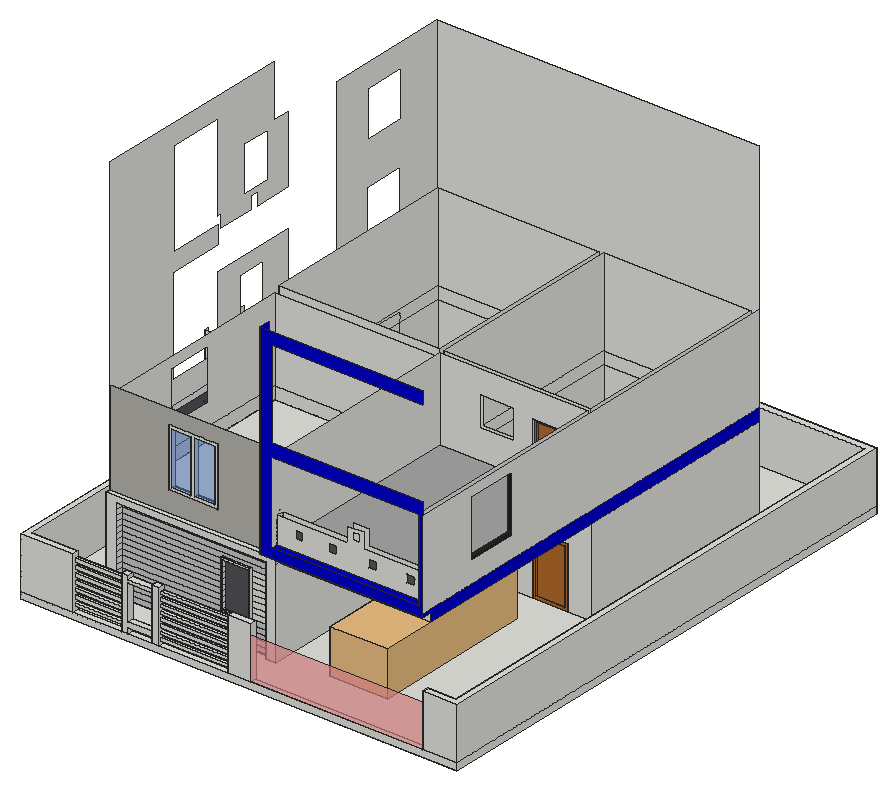
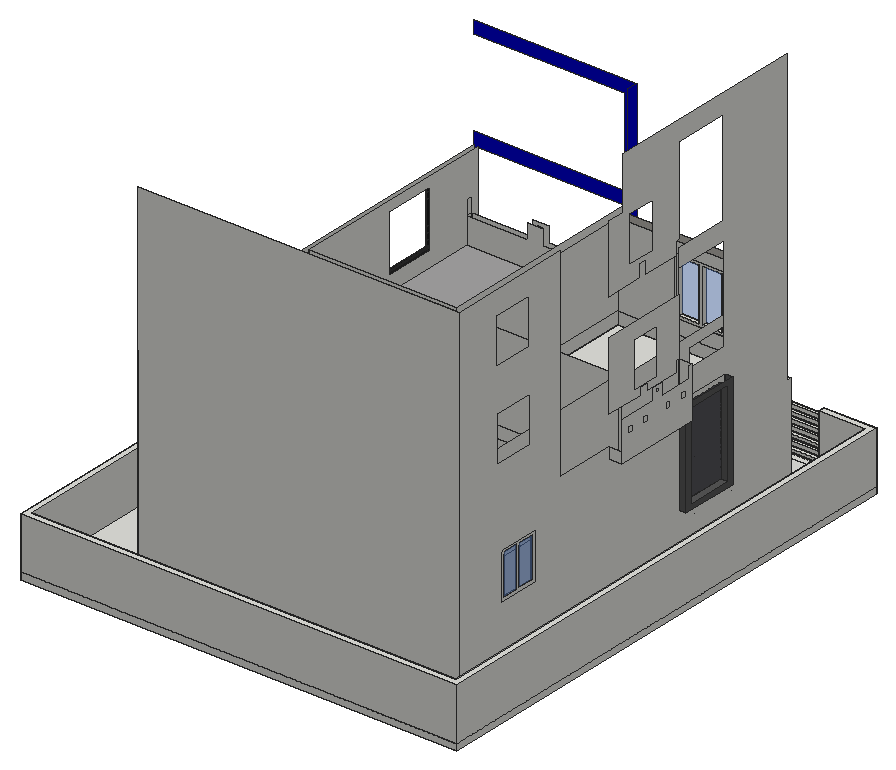
# SketchUp Ruby script. Lengths in inches.
U = 1.inch
M = Sketchup.active_model
def pt(a) = Geom::Point3d.new(a.map { |v| v * U })
def face(e, loops, mat)
  f = e.add_face(loops[0].map { |a| pt(a) })
  loops[1..].each { |l| e.add_face(l.map { |a| pt(a) }).erase! }
  f.material = f.back_material = mat if mat
  f
end
# faces: each face lists its corners as indices into pts; further lists are holes
def faces(e, pts, list, mat = nil) = list.each { |f| face(e, (f[0].is_a?(Array) ? f : [f]).map { |l| l.map { |i| pts[i] } }, mat) }
# xy, xz, yz: faces in a plane at the given z, y or x. An outline is a flat list of corners, or four numbers for a rectangle; further outlines are holes
def ring(l) = l.size == 4 ? [[l[0], l[1]], [l[2], l[1]], [l[2], l[3]], [l[0], l[3]]] : l.each_slice(2).to_a
def flat(e, list, mat, &to3) = list.each { |f| face(e, (f[0].is_a?(Array) ? f : [f]).map { |l| ring(l).map { |u, v| to3.(u, v) } }, mat) }
def xy(e, z, list, mat = nil) = flat(e, list, mat) { |x, y| [x, y, z] }
def xz(e, y, list, mat = nil) = flat(e, list, mat) { |x, z| [x, y, z] }
def yz(e, x, list, mat = nil) = flat(e, list, mat) { |y, z| [x, y, z] }
def lines(e, pts, list) = list.each { |a, b| e.add_line(pt(pts[a]), pt(pts[b])) }
# prism: a flat outline (further loops are holes) pulled along v
def prism(e, loops, v, mat = nil)
  f = face(e, loops, mat); d = Geom::Vector3d.new(v.map { |x| x * U })
  f.pushpull(f.normal.samedirection?(d) ? d.length : -d.length)
end
def box(e, o, s, mat = nil) = prism(e, [[o, [o[0] + s[0], o[1], o[2]], [o[0] + s[0], o[1] + s[1], o[2]], [o[0], o[1] + s[1], o[2]]]], [0, 0, s[2]], mat)
def at(x, y, z, deg = 0) = Geom::Transformation.translation(pt([x, y, z])) * Geom::Transformation.rotation(ORIGIN, Z_AXIS, deg.degrees)
def axes(o, x, y, z) = Geom::Transformation.new([*x, 0, *y, 0, *z, 0, *pt(o).to_a, 1])
def part(name) = M.definitions.add(name)
# library, detail: a bought-in or finely detailed component or shape, given as its bounding box
def library(name, o, s) = part(name).tap { |d| box(d.entities, o, s) }
def detail(e, o, s) = box(e.add_group.entities, o, s)
def put(e, d, t, mat = nil) = e.add_instance(d, t).tap { |i| i.material = mat if mat }
def group(e, t, mat = nil) = e.add_group.tap { |g| g.transformation = t; g.material = mat if mat }.entities
root = M.entities
M.materials.add("[Blinds Roman Hobbled Blue]").color = [81, 82, 87]
M.materials.add("[Color A02]").color = [255, 153, 153]
M.materials["[Color A02]"].alpha = 0.67
M.materials.add("[Color I06]").color = [0, 0, 204]
M.materials.add("[Color M02]").color = [198, 198, 198]
M.materials.add("[Color M06]").color = [86, 86, 86]
M.materials.add("[Color M08]").color = [30, 30, 30]
M.materials.add("[Stone Vein Gray]").color = [166, 165, 165]
M.materials.add("[Tile Travertine 2 inch]").color = [181, 178, 172]
M.materials.add("[Translucent Glass Blue]").color = [100, 149, 237]
M.materials["[Translucent Glass Blue]"].alpha = 0.5
M.materials.add("[Translucent Glass Gray]").color = [128, 128, 128]
M.materials["[Translucent Glass Gray]"].alpha = 0.5
M.materials.add("[Wood Bamboo]").color = [177, 105, 43]
c1 = library("custom el camino",[47.5625,9.86,-8],[222.64,79.59,60.9375])
c2 = part("Group\#1")
xy(c2.entities,0,[[0,0,48,1.5625],[0,1.5625,48,7.5625]],"[Wood Bamboo]")
xy(c2.entities,3.79,[[3.79,0,44.21,1.5625],[3.79,1.5625,44.21,7.5625]],"[Wood Bamboo]")
xy(c2.entities,80.21,[[3.79,0,44.21,1.5625]])
xy(c2.entities,80.21,[[3.79,1.5625,44.21,7.5625]],"[Wood Bamboo]")
xy(c2.entities,84,[[0,0,48,7.5625]],"[Wood Bamboo]")
xz(c2.entities,0,[[[0,0,48,84],[3.79,3.79,44.21,80.21]]],"[Wood Bamboo]")
xz(c2.entities,1.5625,[[3.79,3.79,44.21,80.21]],"[Wood Bamboo]")
xz(c2.entities,7.5625,[[[0,0,48,84],[3.79,3.79,44.21,80.21]],[3.79,3.79,44.21,80.21]],"[Wood Bamboo]")
yz(c2.entities,0,[[0,0,7.5625,84]],"[Wood Bamboo]")
yz(c2.entities,3.79,[[0,3.79,1.5625,80.21],[1.5625,3.79,7.5625,80.21]],"[Wood Bamboo]")
yz(c2.entities,44.21,[[0,3.79,1.5625,80.21],[1.5625,3.79,7.5625,80.21]],"[Wood Bamboo]")
yz(c2.entities,48,[[0,0,7.5625,84]],"[Wood Bamboo]")
c3 = part("Group\#4")
xy(c3.entities,0,[[0,0,32.875,4]])
xy(c3.entities,2.47,[[2.47,0,30.4,4]])
xy(c3.entities,30.4,[[2.47,0,30.4,4]])
xy(c3.entities,32.875,[[0,0,32.875,4]])
xz(c3.entities,0,[[[0,0,32.875,32.875],[2.47,2.47,30.4,30.4]]])
xz(c3.entities,0,[[2.47,2.47,30.4,30.4]],"[Translucent Glass Gray]")
xz(c3.entities,4,[[[0,0,32.875,32.875],[2.47,2.47,30.4,30.4]]])
yz(c3.entities,0,[[0,0,4,32.875]])
yz(c3.entities,2.47,[[0,2.47,4,30.4]])
yz(c3.entities,30.4,[[0,2.47,4,30.4]])
yz(c3.entities,32.875,[[0,0,4,32.875]])
c4 = part("Group\#2")
xy(c4.entities,0,[[0,0,37.8125,5]])
xy(c4.entities,2.57,[[2.57,0,17.37,5],[19.91,0,35.24,5]])
xy(c4.entities,44.8,[[2.57,0,17.37,5],[19.91,0,35.24,5]])
xy(c4.entities,47.375,[[0,0,37.8125,5]])
xz(c4.entities,0,[[[0,0,37.8125,47.375],[19.91,2.57,35.24,44.8],[2.57,2.57,17.37,44.8]]])
xz(c4.entities,0,[[2.57,2.57,17.37,44.8],[19.91,2.57,35.24,44.8]],"[Translucent Glass Blue]")
xz(c4.entities,5,[[[0,0,37.8125,47.375],[19.91,2.57,35.24,44.8],[2.57,2.57,17.37,44.8]]])
yz(c4.entities,0,[[0,0,5,47.375]])
yz(c4.entities,2.57,[[0,2.57,5,44.8]])
yz(c4.entities,17.37,[[0,2.57,5,44.8]])
yz(c4.entities,19.91,[[0,2.57,5,44.8]])
yz(c4.entities,35.24,[[0,2.57,5,44.8]])
yz(c4.entities,37.8125,[[0,0,5,47.375]])
c5 = part("Group\#3")
xy(c5.entities,0,[[0,0,37.8125,5]])
xy(c5.entities,2.57,[[2.57,0,17.37,5],[19.91,0,35.24,5]])
xy(c5.entities,44.8,[[2.57,0,17.37,5],[19.91,0,35.24,5]])
xy(c5.entities,47.375,[[0,0,37.8125,5]])
xz(c5.entities,0,[[[0,0,37.8125,47.375],[19.91,2.57,35.24,44.8],[2.57,2.57,17.37,44.8]]])
xz(c5.entities,0,[[2.57,2.57,17.37,44.8],[19.91,2.57,35.24,44.8]],"[Translucent Glass Blue]")
xz(c5.entities,5,[[[0,0,37.8125,47.375],[19.91,2.57,35.24,44.8],[2.57,2.57,17.37,44.8]]])
yz(c5.entities,0,[[0,0,5,47.375]])
yz(c5.entities,2.57,[[0,2.57,5,44.8]])
yz(c5.entities,17.37,[[0,2.57,5,44.8]])
yz(c5.entities,19.91,[[0,2.57,5,44.8]])
yz(c5.entities,35.24,[[0,2.57,5,44.8]])
yz(c5.entities,37.8125,[[0,0,5,47.375]])
xy(root,0,[[0,0,600,720]])
xy(root,9,[[0,0,0,720,600,720,600,0,552.82,0,552.82,9,591,9,591,711,9,711,9,9,72.1875,9,72.1875,0],[72.1875,0,138.87,9],[138.87,0,147.87,9],[147.87,0,180.05,9],[180.05,0,189.93,9],
  [189.93,0,285.1,9],[285.1,0,316.67,9],[316.67,0,552.82,9],[[9,9,591,711],[77.4375,49.875,77.4375,619.125,518.75,619.125,518.75,332.8125,486.18,332.8125,486.18,338.8125,438.18,338.8125,438.18,332.8125,310.75,332.8125,310.75,49.875,296.85,49.875,296.85,56.875,93.29,56.875,93.29,49.875]],[[77.4375,49.875,77.4375,619.125,518.75,619.125,518.75,332.8125,486.18,332.8125,486.18,338.8125,512.75,338.8125,512.75,613.125,310.75,613.125,310.75,338.8125,438.18,338.8125,438.18,332.8125,310.75,332.8125,310.75,49.875,296.85,49.875,296.85,56.875,93.29,56.875,93.29,49.875],[83.4375,338.8125,304.75,613.125],[83.4375,62.875,304.75,332.8125]],
  [83.4375,62.875,304.75,332.8125],[83.4375,338.8125,304.75,613.125],[310.75,338.8125,512.75,613.125]])
xy(root,14.68,[[189.54,2.77,285.1,7.27]])
xy(root,15.75,[[72.1875,2.58,142.25,7.21]])
xy(root,16.68,[[147.87,0,180,9]])
xy(root,18.49,[[189.54,2.77,285.1,7.27]])
xy(root,20.375,[[72.1875,2.58,142.25,7.21]])
xy(root,22.74,[[189.6,2.93,285.1,7.12]])
xy(root,24.37,[[147.87,0,180,9]])
xy(root,24.875,[[72.1875,2.58,138.5625,7.21]])
xy(root,26.92,[[189.6,2.93,285.1,7.12]])
xy(root,29.5,[[72.1875,2.58,138.5625,7.21]])
xy(root,30.92,[[187.85,2.93,285.1,7.12]])
xy(root,34,[[72.1875,2.58,139.25,7.21]])
xy(root,35.11,[[187.85,2.93,285.1,7.12]])
xy(root,38.625,[[72.1875,2.58,139.25,7.21]])
xy(root,39.11,[[189.85,2.93,285.1,7.12]])
xy(root,43.125,[[72.1875,2.58,139.1875,7.21]])
xy(root,43.3,[[189.85,2.93,285.1,7.12]])
xy(root,43.58,[[232.47,53.1875,272.78,56.875]])
xy(root,45.28,[[235.35,53.1875,271.02,56.875]])
xy(root,47.3,[[189.29,2.93,285.1,7.12]])
xy(root,47.75,[[72.1875,2.58,139.1875,7.21]])
xy(root,51.49,[[189.29,2.93,285.1,7.12]])
xy(root,52.25,[[72.1875,2.58,138.87,7.21]])
xy(root,54.29,[[364.5,332.8125,411.32,338.8125]])
xy(root,55.49,[[189.79,2.93,285.1,7.12]])
xy(root,56.875,[[72.1875,2.58,138.87,7.21]])
xy(root,59.375,[[67.1875,163.22,77.4375,242.75]],"[Color M06]")
xy(root,59.67,[[189.79,2.93,285.1,7.12]])
xy(root,61.375,[[72.1875,2.58,138.625,7.21]])
xy(root,63.67,[[189.93,2.93,285.1,7.12]])
xy(root,66,[[72.1875,2.58,138.625,7.21]])
xy(root,66.7,[[67.1875,170.55,77.4375,235.42]],"[Color M06]")
xy(root,67.86,[[189.93,2.93,285.1,7.12]])
xy(root,70.5,[[72.1875,2.58,138.87,7.21]])
xy(root,71.59,[[147.87,0,180.05,9]])
xy(root,71.86,[[189.35,2.93,285.1,7.12]])
xy(root,75.125,[[72.1875,2.58,138.87,7.21]])
xy(root,76.05,[[189.35,2.93,285.1,7.12]])
xy(root,76.29,[[147.87,0,180.05,9]])
xy(root,80.27,[[77.4375,489.73,83.4375,546.67]])
xy(root,81,[[0,0,72.1875,0,72.1875,9,9,9,9,711,591,711,591,9,552.82,9,552.82,0,600,0,600,720,0,720],[138.87,0,147.87,9],[180.05,0,189.93,9],[285.1,0,316.67,9]])
xy(root,93,[[438.18,332.8125,486.18,338.8125]])
xy(root,95.54,[[364.5,332.8125,411.32,338.8125]])
xy(root,108.26,[[235.35,53.1875,270.98,56.875]])
xy(root,109.97,[[232.47,53.1875,272.68,56.875]])
xy(root,123,[[83.4375,62.875,304.75,332.8125]])
xy(root,129,[[93.29,49.875,296.85,56.875],[310.75,56.875,518.75,332.8125],[83.4375,62.875,304.75,332.8125]])
xy(root,137.25,[[77.4375,49.875,310.75,56.875]])
xy(root,140.25,[[295.25,42.6875,310.75,56.875],[310.75,42.6875,518.75,56.875]])
xy(root,142.7,[[77.4375,489.73,83.4375,546.67]])
xy(root,153.3125,[[310.75,52.875,512.75,62.01]])
xy(root,153.3125,[[310.75,42.6875,512.75,52.875]],"[Color I06]")
xy(root,153.3125,[[310.75,62.01,512.75,62.01,512.75,332.8125,486.18,332.8125,486.18,338.8125,438.18,338.8125,438.18,332.8125,310.75,332.8125]],"[Stone Vein Gray]")
xy(root,164.56,[[157.85,56.875,226.03,62.875]])
xy(root,174.48,[[512.75,125.55,518.75,195.62]],"[Color M08]")
xy(root,175.33,[[59.3125,242.75,77.4375,362.77]])
xz(root,0,[[0,0,600,9],[0,9,72.1875,81],[138.87,9,147.87,9,147.87,16.68,180,16.68,180,24.37,147.87,24.37,147.87,71.59,180.05,71.59,180.05,76.29,147.87,76.29,147.87,81,138.87,81],[180.05,9,189.93,81],[285.1,9,316.67,81],
  [552.82,9,600,81]])
xz(root,0,[[316.67,9,552.82,67.52]],"[Color A02]")
xz(root,2.58,[[72.1875,15.75,142.25,20.375],[72.1875,24.875,138.5625,29.5],[72.1875,34,139.25,38.625],[72.1875,43.125,139.1875,47.75],[72.1875,52.25,138.87,56.875],
  [72.1875,61.375,138.625,66],[72.1875,70.5,138.87,75.125]])
xz(root,2.77,[[189.54,14.68,285.1,18.49]])
xz(root,2.93,[[189.6,22.74,285.1,26.92],[187.85,30.92,285.1,35.11],[189.85,39.11,285.1,43.3],[189.29,47.3,285.1,51.49],[189.79,55.49,285.1,59.67],
  [189.93,63.67,285.1,67.86],[189.35,71.86,285.1,76.05]])
xz(root,7.12,[[189.6,22.74,285.1,26.92],[187.85,30.92,285.1,35.11],[189.85,39.11,285.1,43.3],[189.29,47.3,285.1,51.49],[189.79,55.49,285.1,59.67],
  [189.93,63.67,285.1,67.86],[189.35,71.86,285.1,76.05]])
xz(root,7.21,[[72.1875,15.75,142.25,20.375],[72.1875,24.875,138.5625,29.5],[72.1875,34,139.25,38.625],[72.1875,43.125,139.1875,47.75],[72.1875,52.25,138.87,56.875],
  [72.1875,61.375,138.625,66],[72.1875,70.5,138.87,75.125]])
xz(root,7.27,[[189.54,14.68,285.1,18.49]])
xz(root,9,[[9,9,72.1875,81],[138.87,9,138.87,81,147.87,81,147.87,76.29,180.05,76.29,180.05,71.59,147.87,71.59,147.87,24.37,180,24.37,180,16.68,147.87,16.68,147.87,9],[180.05,9,189.93,81],[285.1,9,316.67,81],[552.82,9,591,81]])
xz(root,42.6875,[[[295.25,140.25,518.75,140.25,518.75,283,310.75,283,310.75,403,518.75,403,518.75,420,295.25,420],[310.75,153.3125,512.75,266]]],"[Color I06]")
xz(root,49.875,[[77.4375,9,93.29,9,93.29,129,296.85,129,296.85,9,310.75,9,310.75,137.25,77.4375,137.25]])
xz(root,52.875,[[[310.75,153.3125,512.75,153.3125,512.75,189.3125,428.93,189.3125,428.93,209.8125,408.29,209.8125,408.29,189.3125,310.75,189.3125],[335.72,169.125,346.47,179.875],[381.1,169.125,391.85,179.875],[436.72,169.125,447.47,179.875],[488.85,169.125,499.6,179.875],[414.09,194.96,423.78,205.53]]])
xz(root,52.875,[[335.72,169.125,346.47,179.875],[381.1,169.125,391.85,179.875],[436.72,169.125,447.47,179.875],[488.85,169.125,499.6,179.875]],"[Color M06]")
xz(root,53.1875,[[[232.47,43.58,272.78,43.58,272.68,46.83,272.68,109.97,232.47,109.97],[235.35,45.28,235.35,108.26,270.98,108.26,270.98,46.8,271.02,45.28]]])
xz(root,56.875,[[93.29,9,296.85,9.33],[[232.47,43.58,232.47,109.97,272.68,109.97,272.68,46.83,272.78,43.58],[235.35,45.28,271.02,45.28,270.98,46.8,270.98,108.26,235.35,108.26]],[272.68,46.83,296.85,54.33],[272.68,54.33,296.85,61.83],[272.68,61.83,296.85,69.33],
  [272.68,69.33,296.85,76.83],[272.68,76.83,296.85,84.33],[272.68,84.33,296.85,91.83],[272.68,91.83,296.85,99.33],[272.68,99.33,296.85,106.83],
  [310.75,129,518.75,140.25]])
xz(root,56.875,[[235.35,45.28,271.02,45.28,270.98,46.8,270.98,108.26,235.35,108.26]],"[Blinds Roman Hobbled Blue]")
xz(root,56.875,[[93.29,9.33,296.85,16.83],[93.29,16.83,296.85,24.33],[93.29,24.33,296.85,31.83],[93.29,31.83,296.85,39.33],[93.29,39.33,296.85,39.33,296.85,46.83,272.68,46.83,272.78,43.58,232.47,43.58,232.47,46.83,93.29,46.83],
  [93.29,46.83,232.47,54.33],[93.29,54.33,232.47,61.83],[93.29,61.83,232.47,69.33],[93.29,69.33,232.47,76.83],[93.29,76.83,232.47,84.33],
  [93.29,84.33,232.47,91.83],[93.29,91.83,232.47,99.33],[93.29,99.33,232.47,106.83],[93.29,106.83,232.47,106.83,232.47,109.97,272.68,109.97,272.68,106.83,296.85,106.83,296.85,114.33,93.29,114.33],[93.29,114.33,296.85,121.83],
  [93.29,121.83,296.85,129]],"[Color M02]")
xz(root,56.875,[[[77.4375,137.25,310.75,137.25,310.75,140.25,295.25,140.25,295.25,266,77.4375,266],[157.85,164.56,226.03,245.87]]],"[Tile Travertine 2 inch]")
xz(root,62.01,[[310.75,153.3125,310.75,189.3125,408.29,189.3125,408.29,209.8125,428.93,209.8125,428.93,189.3125,512.75,189.3125,512.75,153.3125]])
xz(root,62.875,[[83.4375,9,304.75,123],[83.4375,123,304.75,129],[83.4375,129,304.75,146],[[83.4375,146,304.75,260],[157.85,164.56,226.03,245.87]]])
xz(root,125.55,[[515.8,143.44,515.47,143.49,515.17,143.61,514.91,143.81,514.72,144.07,514.59,144.37,514.55,144.69,514.59,145.02,514.72,145.32,514.91,145.58,515.17,145.78,515.47,145.9,515.8,145.94,516.12,145.9,516.42,145.78,516.68,145.58,516.88,145.32,517.01,145.02,517.05,144.69,517.01,144.37,516.88,144.07,516.68,143.81,516.42,143.61,516.12,143.49],[515.8,151.88,515.47,151.92,515.17,152.05,514.91,152.25,514.72,152.51,514.59,152.81,514.55,153.13,514.59,153.45,514.72,153.76,514.91,154.01,515.17,154.21,515.47,154.34,515.8,154.38,516.12,154.34,516.42,154.21,516.68,154.01,516.88,153.76,517.01,153.45,517.05,153.13,517.01,152.81,516.88,152.51,516.68,152.25,516.42,152.05,516.12,151.92],[515.8,160.32,515.47,160.36,515.17,160.49,514.91,160.68,514.72,160.94,514.59,161.24,514.55,161.57,514.59,161.89,514.72,162.19,514.91,162.45,515.17,162.65,515.47,162.78,515.8,162.82,516.12,162.78,516.42,162.65,516.68,162.45,516.88,162.19,517.01,161.89,517.05,161.57,517.01,161.24,516.88,160.94,516.68,160.68,516.42,160.49,516.12,160.36],[515.8,168.76,515.47,168.8,515.17,168.92,514.91,169.12,514.72,169.38,514.59,169.68,514.55,170.01,514.59,170.33,514.72,170.63,514.91,170.89,515.17,171.09,515.47,171.21,515.8,171.26,516.12,171.21,516.42,171.09,516.68,170.89,516.88,170.63,517.01,170.33,517.05,170.01,517.01,169.68,516.88,169.38,516.68,169.12,516.42,168.92,516.12,168.8],[515.8,177.19,516.12,177.24,516.42,177.36,516.68,177.56,516.88,177.82,517.01,178.12,517.05,178.44,517.01,178.77,516.88,179.07,516.68,179.33,516.42,179.53,516.12,179.65,515.8,179.69,515.47,179.65,515.17,179.53,514.91,179.33,514.72,179.07,514.59,178.77,514.55,178.44,514.59,178.12,514.72,177.82,514.91,177.56,515.17,177.36,515.47,177.24]])
xz(root,125.55,[[[512.75,174.48,518.75,253.54],[515.8,244.69,516.12,244.74,516.42,244.86,516.68,245.06,516.88,245.32,517.01,245.62,517.05,245.94,517.01,246.27,516.88,246.57,516.68,246.83,516.42,247.03,516.12,247.15,515.8,247.19,515.47,247.15,515.17,247.03,514.91,246.83,514.72,246.57,514.59,246.27,514.55,245.94,514.59,245.62,514.72,245.32,514.91,245.06,515.17,244.86,515.47,244.74],[515.8,236.26,516.12,236.3,516.42,236.42,516.68,236.62,516.88,236.88,517.01,237.18,517.05,237.51,517.01,237.83,516.88,238.13,516.68,238.39,516.42,238.59,516.12,238.71,515.8,238.76,515.47,238.71,515.17,238.59,514.91,238.39,514.72,238.13,514.59,237.83,514.55,237.51,514.59,237.18,514.72,236.88,514.91,236.62,515.17,236.42,515.47,236.3],[515.8,227.82,516.12,227.86,516.42,227.99,516.68,228.18,516.88,228.44,517.01,228.74,517.05,229.07,517.01,229.39,516.88,229.69,516.68,229.95,516.42,230.15,516.12,230.28,515.8,230.32,515.47,230.28,515.17,230.15,514.91,229.95,514.72,229.69,514.59,229.39,514.55,229.07,514.59,228.74,514.72,228.44,514.91,228.18,515.17,227.99,515.47,227.86],[515.8,219.38,516.12,219.42,516.42,219.55,516.68,219.75,516.88,220.01,517.01,220.31,517.05,220.63,517.01,220.95,516.88,221.26,516.68,221.51,516.42,221.71,516.12,221.84,515.8,221.88,515.47,221.84,515.17,221.71,514.91,221.51,514.72,221.26,514.59,220.95,514.55,220.63,514.59,220.31,514.72,220.01,514.91,219.75,515.17,219.55,515.47,219.42],[515.8,210.94,516.12,210.99,516.42,211.11,516.68,211.31,516.88,211.57,517.01,211.87,517.05,212.19,517.01,212.52,516.88,212.82,516.68,213.08,516.42,213.28,516.12,213.4,515.8,213.44,515.47,213.4,515.17,213.28,514.91,213.08,514.72,212.82,514.59,212.52,514.55,212.19,514.59,211.87,514.72,211.57,514.91,211.31,515.17,211.11,515.47,210.99],[515.8,202.51,516.12,202.55,516.42,202.67,516.68,202.87,516.88,203.13,517.01,203.43,517.05,203.76,517.01,204.08,516.88,204.38,516.68,204.64,516.42,204.84,516.12,204.96,515.8,205.01,515.47,204.96,515.17,204.84,514.91,204.64,514.72,204.38,514.59,204.08,514.55,203.76,514.59,203.43,514.72,203.13,514.91,202.87,515.17,202.67,515.47,202.55],[515.8,194.07,516.12,194.11,516.42,194.24,516.68,194.43,516.88,194.69,517.01,194.99,517.05,195.32,517.01,195.64,516.88,195.94,516.68,196.2,516.42,196.4,516.12,196.53,515.8,196.57,515.47,196.53,515.17,196.4,514.91,196.2,514.72,195.94,514.59,195.64,514.55,195.32,514.59,194.99,514.72,194.69,514.91,194.43,515.17,194.24,515.47,194.11],[515.8,185.63,516.12,185.67,516.42,185.8,516.68,186,516.88,186.26,517.01,186.56,517.05,186.88,517.01,187.2,516.88,187.51,516.68,187.76,516.42,187.96,516.12,188.09,515.8,188.13,515.47,188.09,515.17,187.96,514.91,187.76,514.72,187.51,514.59,187.2,514.55,186.88,514.59,186.56,514.72,186.26,514.91,186,515.17,185.8,515.47,185.67],[515.8,177.19,516.12,177.24,516.42,177.36,516.68,177.56,516.88,177.82,517.01,178.12,517.05,178.44,517.01,178.77,516.88,179.07,516.68,179.33,516.42,179.53,516.12,179.65,515.8,179.69,515.47,179.65,515.17,179.53,514.91,179.33,514.72,179.07,514.59,178.77,514.55,178.44,514.59,178.12,514.72,177.82,514.91,177.56,515.17,177.36,515.47,177.24]]],"[Color M08]")
xz(root,163.22,[[67.1875,59.375,77.4375,192.66]],"[Color M06]")
xz(root,170.55,[[67.1875,66.7,77.4375,185.33]],"[Color M06]")
xz(root,195.62,[[[512.75,174.48,518.75,253.54],[515.8,244.69,515.47,244.74,515.17,244.86,514.91,245.06,514.72,245.32,514.59,245.62,514.55,245.94,514.59,246.27,514.72,246.57,514.91,246.83,515.17,247.03,515.47,247.15,515.8,247.19,516.12,247.15,516.42,247.03,516.68,246.83,516.88,246.57,517.01,246.27,517.05,245.94,517.01,245.62,516.88,245.32,516.68,245.06,516.42,244.86,516.12,244.74],[515.8,236.26,515.47,236.3,515.17,236.42,514.91,236.62,514.72,236.88,514.59,237.18,514.55,237.51,514.59,237.83,514.72,238.13,514.91,238.39,515.17,238.59,515.47,238.71,515.8,238.76,516.12,238.71,516.42,238.59,516.68,238.39,516.88,238.13,517.01,237.83,517.05,237.51,517.01,237.18,516.88,236.88,516.68,236.62,516.42,236.42,516.12,236.3],[515.8,194.07,515.47,194.11,515.17,194.24,514.91,194.43,514.72,194.69,514.59,194.99,514.55,195.32,514.59,195.64,514.72,195.94,514.91,196.2,515.17,196.4,515.47,196.53,515.8,196.57,516.12,196.53,516.42,196.4,516.68,196.2,516.88,195.94,517.01,195.64,517.05,195.32,517.01,194.99,516.88,194.69,516.68,194.43,516.42,194.24,516.12,194.11],[515.8,210.94,515.47,210.99,515.17,211.11,514.91,211.31,514.72,211.57,514.59,211.87,514.55,212.19,514.59,212.52,514.72,212.82,514.91,213.08,515.17,213.28,515.47,213.4,515.8,213.44,516.12,213.4,516.42,213.28,516.68,213.08,516.88,212.82,517.01,212.52,517.05,212.19,517.01,211.87,516.88,211.57,516.68,211.31,516.42,211.11,516.12,210.99]]],"[Color M08]")
xz(root,196.24,[[515.8,177.19,515.47,177.24,515.17,177.36,514.91,177.56,514.72,177.82,514.59,178.12,514.55,178.44,514.59,178.77,514.72,179.07,514.91,179.33,515.17,179.53,515.47,179.65,515.8,179.69,516.12,179.65,516.42,179.53,516.68,179.33,516.88,179.07,517.01,178.77,517.05,178.44,517.01,178.12,516.88,177.82,516.68,177.56,516.42,177.36,516.12,177.24]])
xz(root,235.42,[[67.1875,66.7,77.4375,185.33]],"[Color M06]")
xz(root,242.75,[[59.3125,175.33,67.1875,175.33,67.1875,192.66,77.4375,192.66,77.4375,246.02,59.3125,246.02],[67.1875,175.33,77.4375,192.66]])
xz(root,242.75,[[67.1875,59.375,77.4375,175.33]],"[Color M06]")
xz(root,332.8125,[[83.4375,9,304.75,123],[[310.75,9,438.18,9,438.18,93,486.18,93,486.18,9,518.75,9,518.75,129,310.75,129],[364.5,54.29,411.32,95.54]],[83.4375,123,194.09,129],[194.09,123,222.91,129],[222.91,123,304.75,129],
  [83.4375,129,304.75,146],[83.4375,146,304.75,260],[[310.75,153.3125,438.18,153.3125,438.18,230,486.18,230,486.18,153.3125,512.75,153.3125,512.75,266,310.75,266],[364.5,192.97,411.32,234.22]]])
xz(root,338.8125,[[83.4375,9,304.75,129],[[310.75,9,310.75,129,512.75,129,512.75,9,486.18,9,486.18,93,438.18,93,438.18,9],[364.5,54.29,411.32,95.54]],[83.4375,129,304.75,146],[310.75,129,310.75,146,438.18,146,438.18,153.3125,486.18,153.3125,486.18,146,512.75,146,512.75,129],[83.4375,146,304.75,266],
  [[310.75,146,310.75,266,512.75,266,512.75,146,486.18,146,486.18,230,438.18,230,438.18,146],[364.5,192.97,411.32,234.22]]])
xz(root,362.77,[[59.3125,175.33,77.4375,190.375]])
xz(root,489.73,[[77.4375,80.27,83.4375,142.7]])
xz(root,546.67,[[77.4375,80.27,83.4375,142.7]])
xz(root,613.125,[[83.4375,9,304.75,129],[310.75,9,512.75,129],[83.4375,129,304.75,146],[310.75,129,512.75,146],[83.4375,146,304.75,266],
  [310.75,146,512.75,266]])
xz(root,619.125,[[77.4375,9,518.75,468]])
xz(root,711,[[9,9,591,81]])
xz(root,720,[[0,0,600,9],[0,9,600,81]])
yz(root,0,[[0,0,720,9],[0,9,720,81]])
yz(root,9,[[9,9,711,81]])
yz(root,59.3125,[[[242.75,175.33,242.75,246.02,248.07,246.02,248.07,230.24,294.97,229.95,294.97,246.02,309.77,246.02,309.77,229.95,362.77,230.24,362.77,175.33],[344.8125,208.79,353.375,217.35],[318.6875,208.79,327.25,217.35],[279.625,208.79,288.1875,217.35],[253.3125,209.47,261.875,218.03],[300.15,237.48,305.34,242.66]]])
yz(root,67.1875,[[[163.22,59.375,242.75,192.66],[170.55,66.7,235.42,185.33]]],"[Color M06]")
yz(root,72.1875,[[[0,9,9,81],[2.58,70.5,7.21,75.125],[2.58,61.375,7.21,66],[2.58,52.25,7.21,56.875],[2.58,43.125,7.21,47.75],[2.58,34,7.21,38.625],[2.58,24.875,7.21,29.5],[2.58,15.75,7.21,20.375]]])
yz(root,77.4375,[[[49.875,9,49.875,137.25,56.875,137.25,56.875,540,338.8125,540,338.8125,468,362.77,468,362.77,375.04,311.55,375.04,311.55,392.36,298.6,392.36,298.6,375.04,248.07,375.04,248.07,392.36,241.87,392.36,241.87,512.67,166.06,512.67,166.06,382.11,241.6875,382.11,241.6875,356.84,164.28,356.84,164.28,225.6875,241.6875,225.6875,241.6875,323.97,362.77,323.97,362.77,230.24,309.77,229.95,309.77,246.02,294.97,246.02,294.97,229.95,248.07,230.24,248.07,246.02,242.75,246.02,242.75,192.66,163.22,192.66,163.22,59.375,242.75,59.375,242.75,175.33,362.77,175.33,362.77,190.375,446.27,190.375,446.27,468,619.125,468,619.125,9],[498.5625,252.44,555.5,314.88],[500.02,373.64,556.96,436.08],[489.73,80.27,546.67,142.7],[287.71,398.88,327.77,461.44],[279.8125,240.34,319.875,302.91]],[[163.22,59.375,242.75,192.66],[170.55,66.7,235.42,185.33]]])
yz(root,77.4375,[[170.55,66.7,235.42,185.33]],"[Blinds Roman Hobbled Blue]")
yz(root,83.4375,[[62.875,9,332.8125,123],[338.8125,9,613.125,9,613.125,129,546.67,129,546.67,80.27,489.73,80.27,489.73,129,338.8125,129],[489.73,80.27,546.67,129],[62.875,123,332.8125,129],[62.875,129,332.8125,146],
  [338.8125,129,489.73,129,489.73,142.7,546.67,142.7,546.67,129,613.125,129,613.125,146,338.8125,146],[489.73,129,546.67,142.7],[[62.875,146,332.8125,260],[153.86,176.04,217.18,245.85]],[338.8125,146,613.125,266]])
yz(root,93.29,[[49.875,9,56.875,9.33],[49.875,9.33,56.875,16.83],[49.875,16.83,56.875,24.33],[49.875,24.33,56.875,31.83],[49.875,31.83,56.875,39.33],
  [49.875,39.33,56.875,46.83],[49.875,46.83,56.875,54.33],[49.875,54.33,56.875,61.83],[49.875,61.83,56.875,69.33],[49.875,69.33,56.875,76.83],
  [49.875,76.83,56.875,84.33],[49.875,84.33,56.875,91.83],[49.875,91.83,56.875,99.33],[49.875,99.33,56.875,106.83],[49.875,106.83,56.875,114.33],
  [49.875,114.33,56.875,121.83],[49.875,121.83,56.875,129]])
yz(root,138.5625,[[2.58,24.875,7.21,29.5]])
yz(root,138.625,[[2.58,61.375,7.21,66]])
yz(root,138.87,[[[0,9,9,81],[2.58,70.5,7.21,75.125],[2.58,52.25,7.21,56.875]]])
yz(root,139.1875,[[2.58,43.125,7.21,47.75]])
yz(root,139.25,[[2.58,34,7.21,38.625]])
yz(root,142.25,[[2.58,15.75,7.21,20.375]])
yz(root,147.87,[[0,9,9,16.68],[0,24.37,9,71.59],[0,76.29,9,81]])
yz(root,157.85,[[56.875,164.56,62.875,245.87]])
yz(root,180,[[0,16.68,9,24.37]])
yz(root,180.05,[[0,9,9,71.59],[0,71.59,9,76.29],[0,76.29,9,81]])
yz(root,187.85,[[2.93,30.92,7.12,35.11]])
yz(root,189.29,[[2.93,47.3,7.12,51.49]])
yz(root,189.35,[[2.93,71.86,7.12,76.05]])
yz(root,189.54,[[2.77,14.68,7.27,18.49]])
yz(root,189.6,[[2.93,22.74,7.12,26.92]])
yz(root,189.79,[[2.93,55.49,7.12,59.67]])
yz(root,189.85,[[2.93,39.11,7.12,43.3]])
yz(root,189.93,[[[0,9,9,81],[2.93,63.67,7.12,67.86]]])
yz(root,226.03,[[56.875,164.56,62.875,245.87]])
yz(root,232.47,[[53.1875,43.58,56.875,109.97]])
yz(root,235.35,[[53.1875,45.28,56.875,46.83],[53.1875,46.83,56.875,54.33],[53.1875,54.33,56.875,61.83],[53.1875,61.83,56.875,69.33],[53.1875,69.33,56.875,76.83],
  [53.1875,76.83,56.875,84.33],[53.1875,84.33,56.875,91.83],[53.1875,91.83,56.875,99.33],[53.1875,99.33,56.875,106.83],[53.1875,106.83,56.875,108.26]])
yz(root,270.98,[[53.1875,46.8,56.875,106.83],[53.1875,106.83,56.875,108.26]])
yz(root,272.68,[[53.1875,46.83,56.875,109.97]])
yz(root,285.1,[[[0,9,9,81],[2.93,71.86,7.12,76.05],[2.93,63.67,7.12,67.86],[2.93,55.49,7.12,59.67],[2.93,47.3,7.12,51.49],[2.93,39.11,7.12,43.3],[2.93,30.92,7.12,35.11],[2.93,22.74,7.12,26.92],[2.77,14.68,7.27,18.49]]])
yz(root,295.25,[[42.6875,140.25,56.875,420]],"[Color I06]")
yz(root,296.85,[[49.875,9,56.875,9.33],[49.875,9.33,56.875,129]])
yz(root,304.75,[[62.875,9,332.8125,123],[338.8125,9,613.125,129],[62.875,123,332.8125,129],[62.875,129,332.8125,146],[338.8125,129,613.125,146],
  [62.875,146,332.8125,260],[338.8125,146,613.125,266]])
yz(root,310.75,[[49.875,9,332.8125,129],[338.8125,9,613.125,129],[49.875,129,56.875,137.25],[338.8125,129,613.125,146],[338.8125,146,613.125,266],
  [[42.6875,153.3125,52.875,153.3125,52.875,189.3125,62.01,189.3125,62.01,153.3125,332.8125,153.3125,332.8125,266,42.6875,266],[56.1,191.91,59.54,195.34]],[52.875,153.3125,62.01,189.3125]])
yz(root,316.67,[[0,9,9,81]])
yz(root,364.5,[[332.8125,54.29,338.8125,95.54]])
yz(root,411.32,[[332.8125,54.29,338.8125,95.54]])
yz(root,438.18,[[332.8125,9,338.8125,93],[332.8125,153.3125,338.8125,230]])
yz(root,486.18,[[332.8125,9,338.8125,93],[332.8125,153.3125,338.8125,230]])
yz(root,512.75,[[338.8125,9,613.125,129],[338.8125,129,613.125,146],[338.8125,146,613.125,266],[[42.6875,153.3125,42.6875,266,332.8125,266,332.8125,153.3125,62.01,153.3125,62.01,189.3125,62.375,209.8125,52.875,209.8125,52.875,153.3125],[125.55,174.48,195.62,253.54]],[52.875,153.3125,62.01,189.3125]])
yz(root,518.75,[[332.8125,9,619.125,129],[[42.6875,146,619.125,266],[125.55,174.48,195.62,253.54]]])
yz(root,518.75,[[56.875,129,619.125,129,619.125,146,42.6875,146,42.6875,140.25,56.875,140.25]],"[Color I06]")
yz(root,552.82,[[0,9,9,81]])
yz(root,591,[[9,9,711,81]])
yz(root,600,[[0,0,720,9],[0,9,720,81]])
p = [[272.78,56.875,43.58],[272.68,56.875,46.83],[272.68,53.1875,46.83],[272.78,53.1875,43.58],[270.98,56.875,46.8],[271.02,56.875,45.28],
  [271.02,53.1875,45.28],[270.98,53.1875,46.8],[515.47,125.55,177.24],[515.17,125.55,177.36],[515.17,196.24,177.36],[515.47,196.24,177.24],
  [515.8,125.55,177.19],[515.8,196.24,177.19],[516.12,125.55,177.24],[516.12,196.24,177.24],[516.42,125.55,177.36],[516.42,196.24,177.36],
  [514.91,125.55,177.56],[514.91,196.24,177.56],[516.68,125.55,177.56],[516.68,196.24,177.56],[514.72,125.55,177.82],[514.72,196.24,177.82],
  [516.88,125.55,177.82],[516.88,196.24,177.82],[514.59,125.55,178.12],[514.59,196.24,178.12],[517.01,125.55,178.12],[517.01,196.24,178.12],
  [514.55,125.55,178.44],[514.55,196.24,178.44],[517.05,125.55,178.44],[517.05,196.24,178.44],[514.59,125.55,178.77],[514.59,196.24,178.77],
  [517.01,125.55,178.77],[517.01,196.24,178.77],[514.72,125.55,179.07],[514.72,196.24,179.07],[516.88,125.55,179.07],[516.88,196.24,179.07],
  [514.91,125.55,179.33],[514.91,196.24,179.33],[516.68,125.55,179.33],[516.68,196.24,179.33],[515.17,125.55,179.53],[515.17,196.24,179.53],
  [516.42,125.55,179.53],[516.42,196.24,179.53],[515.47,125.55,179.65],[515.47,196.24,179.65],[516.12,125.55,179.65],[516.12,196.24,179.65],
  [515.8,125.55,179.69],[515.8,196.24,179.69],[77.4375,153.86,176.04],[83.4375,153.86,176.04],[77.4375,217.18,176.04],[83.4375,217.18,176.04],
  [83.4375,216.26,43.875],[83.4375,152.94,43.875],[83.4375,152.94,113.6875],[83.4375,216.26,113.6875],[77.4375,152.94,43.875],[77.4375,216.26,43.875],
  [77.4375,152.94,113.6875],[77.4375,216.26,113.6875]]
faces(root,p,[[0,1,2,3],[4,5,6,7]])
faces(root,p,[[8,9,10,11],[12,8,11,13],[14,12,13,15],[16,14,15,17],[9,18,19,10],[20,16,17,21],[18,22,23,19],[24,20,21,25],
  [22,26,27,23],[28,24,25,29],[26,30,31,27],[32,28,29,33],[30,34,35,31],[36,32,33,37],[34,38,39,35],[40,36,37,41],
  [38,42,43,39],[44,40,41,45],[42,46,47,43],[48,44,45,49],[46,50,51,47],[52,48,49,53],[50,54,55,51],[54,52,53,55]],"[Color M08]")
lines(root,p,[[56,57],[58,59],[60,61],[62,63],[63,60],[64,61],[65,60],[66,62],[67,63]])
put(root,c1,at(463.26,16.35,16.86,90))
put(root,c2,at(438.18,332.8125,9))
put(root,c3,axes([364.63,332.8125,54.29],[1.42,0,0],[0,1,0],[0,0,1.25475]))
put(root,c4,axes([77.33,546.67,80.27],[0,-1.50579,0],[0.41,0,0],[0,0,1.32058]))
put(root,c2,axes([438.17,334.85,153.3125],[1.0001,0,0],[0,0.73,0],[0,0,0.9198]))
put(root,c5,axes([157.85,56.875,164.56],[1.80331,0,0],[0,1,0],[0,0,1.71636]))
